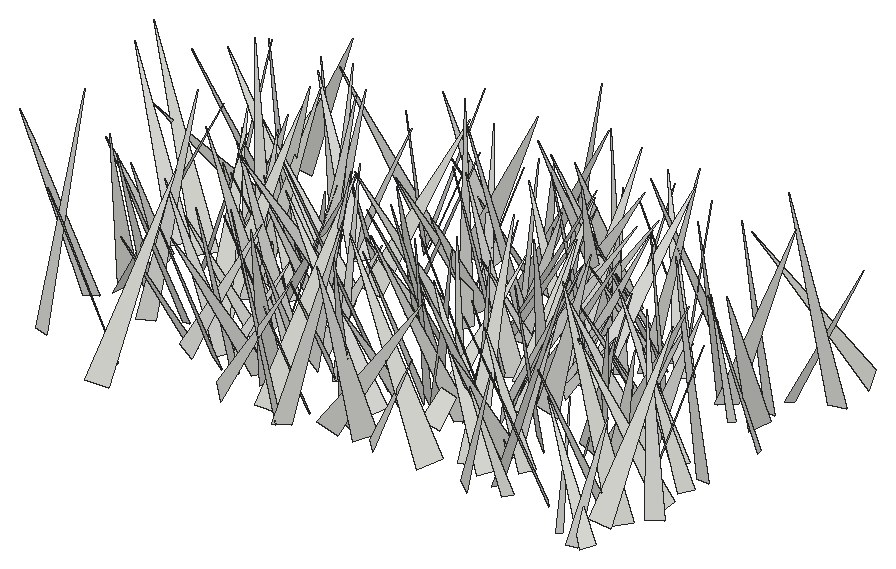
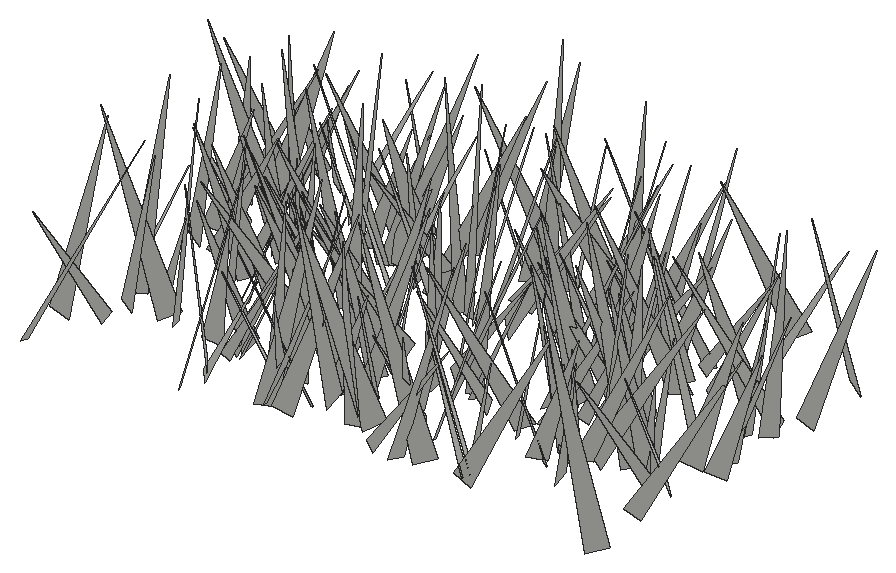
# SketchUp Ruby script. Lengths in inches.
U = 1.inch
M = Sketchup.active_model
def pt(a) = Geom::Point3d.new(a.map { |v| v * U })
def face(e, loops, mat)
  f = e.add_face(loops[0].map { |a| pt(a) })
  loops[1..].each { |l| e.add_face(l.map { |a| pt(a) }).erase! }
  f.material = f.back_material = mat if mat
  f
end
# faces: each face lists its corners as indices into pts; further lists are holes
def faces(e, pts, list, mat = nil) = list.each { |f| face(e, (f[0].is_a?(Array) ? f : [f]).map { |l| l.map { |i| pts[i] } }, mat) }
# xy, xz, yz: faces in a plane at the given z, y or x. An outline is a flat list of corners, or four numbers for a rectangle; further outlines are holes
def ring(l) = l.size == 4 ? [[l[0], l[1]], [l[2], l[1]], [l[2], l[3]], [l[0], l[3]]] : l.each_slice(2).to_a
def flat(e, list, mat, &to3) = list.each { |f| face(e, (f[0].is_a?(Array) ? f : [f]).map { |l| ring(l).map { |u, v| to3.(u, v) } }, mat) }
def xy(e, z, list, mat = nil) = flat(e, list, mat) { |x, y| [x, y, z] }
def xz(e, y, list, mat = nil) = flat(e, list, mat) { |x, z| [x, y, z] }
def yz(e, x, list, mat = nil) = flat(e, list, mat) { |y, z| [x, y, z] }
def lines(e, pts, list) = list.each { |a, b| e.add_line(pt(pts[a]), pt(pts[b])) }
# prism: a flat outline (further loops are holes) pulled along v
def prism(e, loops, v, mat = nil)
  f = face(e, loops, mat); d = Geom::Vector3d.new(v.map { |x| x * U })
  f.pushpull(f.normal.samedirection?(d) ? d.length : -d.length)
end
def box(e, o, s, mat = nil) = prism(e, [[o, [o[0] + s[0], o[1], o[2]], [o[0] + s[0], o[1] + s[1], o[2]], [o[0], o[1] + s[1], o[2]]]], [0, 0, s[2]], mat)
def at(x, y, z, deg = 0) = Geom::Transformation.translation(pt([x, y, z])) * Geom::Transformation.rotation(ORIGIN, Z_AXIS, deg.degrees)
def axes(o, x, y, z) = Geom::Transformation.new([*x, 0, *y, 0, *z, 0, *pt(o).to_a, 1])
def part(name) = M.definitions.add(name)
# library, detail: a bought-in or finely detailed component or shape, given as its bounding box
def library(name, o, s) = part(name).tap { |d| box(d.entities, o, s) }
def detail(e, o, s) = box(e.add_group.entities, o, s)
def put(e, d, t, mat = nil) = e.add_instance(d, t).tap { |i| i.material = mat if mat }
def group(e, t, mat = nil) = e.add_group.tap { |g| g.transformation = t; g.material = mat if mat }.entities
root = M.entities
c1 = part("fur_instance\#9")
p = [[0.8125,0,1.79],[0.67,-0.02,1.48],[0,-0.11,0],[0,0.11,0]]
faces(c1.entities,p,[[0,1,2,3]])
put(root,c1,axes([479.78,414.29,-21.66],[5.20163,-5.29224,1.8402],[-4.95757,-5.51713,-1.85336],[-2.61089,-0.0677,7.18539]))
put(root,c1,axes([461.92,409.04,-21.66],[-4.61251,5.93847,1.25396],[5.3205,4.71401,-2.75381],[2.92064,0.79104,6.99694]))
put(root,c1,axes([478.12,414.66,-21.66],[-1.25565,-8.18969,1.33935],[-8.04493,1.53362,1.83538],[2.03567,1.00923,8.07955]))
put(root,c1,axes([461.29,411.97,-21.66],[-4.82792,-3.85999,0.34861],[-3.62589,4.30173,-2.58417],[-1.36894,2.21934,5.6152]))
put(root,c1,axes([468.7,413.11,-21.66],[4.45492,4.83666,0.95124],[4.56601,-3.56591,-3.25273],[1.85733,-2.83468,5.71483]))
put(root,c1,axes([488.74,413.21,-21.66],[3.06956,3.90435,1.71137],[4.25532,-2.68017,-1.51785],[0.25498,-2.27325,4.72887]))
put(root,c1,axes([499.9,412,-21.66],[-3.00277,4.1066,0.06153],[3.92812,2.84936,1.52829],[-1.19912,-0.94951,4.85234]))
put(root,c1,axes([474.04,412.49,-21.66],[-6.46812,-3.13785,1.21731],[-3.3431,6.29489,-1.53709],[0.38946,1.92167,7.02282]))
put(root,c1,axes([466.18,416.07,-21.66],[-2.99336,-6.46525,0.18966],[-6.30073,2.9619,1.52434],[1.46161,-0.47255,6.9596]))
put(root,c1,axes([499.04,411.47,-21.66],[-3.77654,1.99621,0.89861],[1.50689,3.67022,-1.82025],[1.58796,1.26459,3.86442]))
put(root,c1,axes([477.2,413.66,-21.66],[3.63581,-6.29578,1.08718],[-5.74464,-2.67402,3.72648],[2.79605,2.69271,6.24254]))
put(root,c1,axes([480.76,413.72,-21.66],[2.90459,3.11145,0.76807],[3.13189,-2.53582,-1.57117],[0.67994,-1.61126,3.9559]))
put(root,c1,axes([470.27,416.52,-21.66],[7.22069,-3.00234,1.05262],[-2.62839,-7.10035,-2.22196],[-1.79266,-1.6827,7.49769]))
put(root,c1,axes([491.67,414.07,-21.66],[-1.39517,3.65073,1.37856],[3.73252,0.82124,1.60268],[-1.13865,-1.78115,3.56451]))
put(root,c1,axes([485.2,414.16,-21.66],[-7.15301,3.97515,0.71331],[4.02795,6.91641,1.848],[-0.2937,-1.95899,7.97197]))
put(root,c1,axes([469.38,416.59,-21.66],[1.60402,-6.13136,0.73735],[-5.58582,-1.76536,-2.52831],[-2.63361,0.00991,5.81155]))
put(root,c1,axes([497.26,412.36,-21.66],[1.37607,4.21587,0.41156],[3.82506,-1.42264,1.78368],[-1.81985,0.19763,4.06025]))
put(root,c1,axes([494.35,414.9,-21.66],[-5.23491,-4.53939,0.15815],[-4.43832,5.06084,-1.65066],[-0.96564,1.34804,6.72946]))
put(root,c1,axes([474.78,414.67,-21.66],[-4.9499,-5.12629,0.49866],[-4.98162,4.58947,-2.26921],[-1.30806,1.92014,6.75508]))
put(root,c1,axes([474.51,412.32,-21.66],[6.67924,-1.26552,2.75336],[-2.18749,-6.62541,2.26131],[-2.097,2.88046,6.41095]))
put(root,c1,axes([498.57,415.85,-21.66],[-1.67937,-5.43767,0.87836],[-5.25266,1.30456,-1.96667],[-1.65811,1.37475,5.34049]))
put(root,c1,axes([454.89,412.18,-21.66],[3.59561,7.30217,1.1805],[7.09033,-3.77639,1.76345],[-2.10771,-0.24675,7.94609]))
put(root,c1,axes([488.53,418.25,-21.66],[5.3138,-2.81187,1.14067],[-1.98861,-4.96443,-2.9739],[-2.29198,-2.2118,5.22484]))
put(root,c1,axes([488.16,417.92,-21.66],[-0.28332,-7.79704,0.77926],[-7.68212,0.12267,-1.56569],[-1.54472,0.82004,7.64347]))
put(root,c1,axes([463.92,416.53,-21.66],[-1.49578,-4.28811,0.26565],[-3.87905,1.22698,-2.03551],[-1.84701,0.89578,4.0598]))
put(root,c1,axes([478.81,419.45,-21.66],[-5.2943,-3.28141,1.0592],[-2.29433,4.80125,3.40634],[2.57403,-2.46971,5.21479]))
put(root,c1,axes([472.74,419.83,-21.66],[-3.72735,-5.65721,0.3773],[-4.71825,3.34531,3.54775],[3.14396,-1.68653,5.77153]))
put(root,c1,axes([467.91,415.76,-21.66],[-2.85535,-4.62994,1.75531],[-4.89429,2.33192,-1.81068],[-0.75056,2.40755,5.12941]))
put(root,c1,axes([488.83,415.6,-21.66],[-4.99082,4.3261,0.4502],[4.29852,4.80129,1.51542],[-0.66378,-1.43477,6.4286]))
put(root,c1,axes([499.73,415.64,-21.66],[-2.9065,7.574,1.65107],[7.44857,2.24028,2.83534],[-2.14716,-2.4809,7.60092]))
put(root,c1,axes([471.26,418.73,-21.66],[-5.10979,-2.8974,1.28802],[-2.4355,5.15064,1.92434],[2.03034,-1.11347,5.54994]))
put(root,c1,axes([463.72,415.92,-21.66],[1.55014,5.60518,1.20615],[5.3228,-0.94254,-2.46072],[2.13086,-1.72318,5.26933]))
put(root,c1,axes([466.02,417.1875,-21.66],[-3.70212,4.89762,1.86065],[5.19102,3.12087,2.11373],[-0.70854,-2.72541,5.76407]))
put(root,c1,axes([454.44,417.83,-21.66],[-0.79345,-6.87819,1.77521],[-6.83318,0.25089,-2.08208],[-1.94125,1.92821,6.60333]))
put(root,c1,axes([490.68,417.3,-21.66],[-3.29735,3.76242,1.32483],[3.9802,2.99017,1.41439],[-0.2628,-1.92005,4.79874]))
put(root,c1,axes([498.5625,414.88,-21.66],[-1.75958,6.89289,0.89816],[6.66639,1.93582,-1.79628],[1.96924,-0.39424,6.88342]))
put(root,c1,axes([472.59,413.27,-21.66],[-6.00676,5.62271,0.83771],[4.81686,5.68135,-3.59416],[3.01902,2.12255,7.40122]))
put(root,c1,axes([490.35,414.62,-21.66],[7.12647,2.20024,1.82821],[1.44023,-6.99989,2.8102],[-2.47167,2.26505,6.90872]))
put(root,c1,axes([500.64,419.2,-21.66],[-6.49837,1.01991,0.13564],[1.01971,6.26851,1.71854],[-0.13717,-1.71841,6.34946]))
put(root,c1,axes([483.36,419.9375,-21.66],[0.24896,-7.3468,1.55373],[-6.97419,-0.80255,-2.67734],[-2.78393,1.35351,6.84612]))
put(root,c1,axes([468.35,418.7,-21.66],[-2.5232,4.5633,1.53247],[4.25008,1.29942,3.12842],[-2.26029,-2.65076,4.17172]))
put(root,c1,axes([466.23,417.38,-21.66],[1.55212,3.88569,0.28277],[3.69063,-1.36892,-1.44671],[1.24813,-0.78428,3.92616]))
put(root,c1,axes([479.39,420.81,-21.66],[-5.06426,-4.56399,0.84014],[-4.29824,5.08189,1.69768],[1.74956,-0.72593,6.60262]))
put(root,c1,axes([478.31,417.26,-21.66],[-3.77529,6.85051,0.02559],[5.94676,3.26269,3.89536],[-3.40091,-1.89957,6.78296]))
put(root,c1,axes([480.08,420.4,-21.66],[-3.33298,-6.74445,1.96036],[-6.484,3.7887,2.01069],[2.69971,0.77298,7.24938]))
put(root,c1,axes([461.41,418.87,-21.66],[-3.32714,-4.87132,0.7615],[-4.7527,2.92423,-2.05917],[-1.31203,1.7603,5.52806]))
put(root,c1,axes([489.04,420.68,-21.66],[-3.9717,-6.10655,1.7462],[-5.81347,4.32471,1.90107],[2.55787,0.34722,7.03209]))
put(root,c1,axes([488.62,418.5,-21.66],[-0.11529,-4.79427,2.44231],[-5.06003,0.9271,1.58106],[1.8292,2.26244,4.52754]))
put(root,c1,axes([480.81,420.27,-21.66],[7.66875,0.29762,1.40281],[0.64374,-7.5341,-1.92071],[-1.28143,-2.00373,7.43029]))
put(root,c1,axes([455.2,420.63,-21.66],[6.33398,-2.31725,1.64534],[-1.9481,-6.46653,-1.60778],[-2.06922,-1.00519,6.55011]))
put(root,c1,axes([456.36,421.3125,-21.66],[6.05103,1.03829,2.78411],[2.19851,-5.8136,-2.61017],[-1.99898,-3.2509,5.55698]))
put(root,c1,axes([501.05,417.45,-21.66],[-0.8728,6.82324,1.17968],[6.78553,0.6058,1.51645],[-1.38016,-1.33658,6.7096]))
put(root,c1,axes([486.65,419.37,-21.66],[-5.69424,-4.56861,0.52497],[-4.47673,5.31586,-2.29625],[-1.05201,2.10752,6.92992]))
put(root,c1,axes([493.01,421.88,-21.66],[-1.64763,-7.14584,1.34901],[-6.49832,2.06763,3.01567],[3.26416,0.50931,6.68457]))
put(root,c1,axes([466.42,421.19,-21.66],[-7.9399,0.37328,2.34081],[0.92834,8.01881,1.87016],[2.18103,-2.05426,7.72553]))
put(root,c1,axes([487.23,415.73,-21.66],[-7.03666,4.34174,0.35439],[3.96979,6.66848,-2.87454],[1.79361,2.2741,7.75256]))
put(root,c1,axes([491.99,421.95,-21.66],[0.44147,-7.17503,0.62576],[-6.54369,-0.13768,3.03788],[3.00878,0.75334,6.51516]))
put(root,c1,axes([471.04,419.7,-21.66],[-2.12698,-6.60371,3.80122],[-7.1046,3.14508,1.48842],[2.75369,3.0136,6.77625]))
put(root,c1,axes([477.26,419.98,-21.66],[-5.76145,-5.93812,0.42997],[-5.44241,5.01036,-3.73055],[-2.41379,2.87671,7.38502]))
put(root,c1,axes([468.77,420.61,-21.66],[-0.03383,-6.90938,2.82252],[-7.12958,-0.80509,-2.05628],[-2.20801,2.70547,6.5964]))
put(root,c1,axes([485.42,418.86,-21.66],[-5.55203,-0.57439,2.02149],[-1.15794,5.60149,-1.58866],[1.75372,1.88009,5.3508]))
put(root,c1,axes([494.51,421.6,-21.66],[1.53942,-5.44162,0.89342],[-5.38829,-1.28703,1.44538],[1.17292,1.22946,5.46735]))
put(root,c1,axes([459.17,417.55,-21.66],[-6.96616,2.88196,1.8212],[2.05018,6.85162,-3.00033],[2.72382,2.21349,6.91601]))
put(root,c1,axes([493.77,421.69,-21.66],[6.6749,-4.96789,0.00129],[-4.8195,-6.47499,2.02019],[1.20515,1.62135,8.07174]))
put(root,c1,axes([463.91,418.66,-21.66],[-5.45003,5.37343,0.92209],[5.18096,5.51046,-1.48977],[1.69756,0.43353,7.50714]))
put(root,c1,axes([482.04,418.16,-21.66],[-1.93127,6.17376,0.09606],[5.65668,1.80943,-2.5656],[2.47519,0.68189,5.93825]))
put(root,c1,axes([500.32,421.61,-21.66],[-2.9134,4.03937,1.46912],[4.26943,2.51447,1.5531],[-0.49677,-2.07934,4.73205]))
put(root,c1,axes([484.7,422.12,-21.66],[7.11507,4.33314,0.48127],[4.20256,-6.57141,-2.9643],[1.16029,-2.76992,7.78545]))
put(root,c1,axes([470.51,421.43,-21.66],[0.36945,4.73641,1.83647],[4.53767,0.52011,-2.25427],[2.28381,-1.79961,4.18191]))
put(root,c1,axes([455.34,419.4,-21.66],[7.33228,1.89466,0.16833],[1.78282,-7.07911,2.02191],[-0.66303,1.91751,7.29821]))
put(root,c1,axes([477.05,425.04,-21.66],[-6.01376,-4.74049,2.00405],[-3.98095,6.23797,2.80955],[3.26197,-1.12665,7.12348]))
put(root,c1,axes([473.85,419,-21.66],[2.20032,6.76237,0.49836],[6.15454,-2.21163,2.83722],[-2.84601,0.44546,6.52083]))
put(root,c1,axes([463.13,419.77,-21.66],[-0.97355,8.05143,1.14446],[7.84551,1.23329,-2.00251],[2.14086,-0.85824,7.85896]))
put(root,c1,axes([498.41,419.92,-21.66],[4.22042,3.02936,0.44277],[2.70703,-4.0447,1.87014],[-1.43005,1.2839,4.84681]))
put(root,c1,axes([495.32,423.91,-21.66],[-6.50951,0.22142,0.60358],[0.38251,6.26967,1.82536],[0.51674,-1.85181,6.25226]))
put(root,c1,axes([483.3,420.03,-21.66],[5.52585,4.05046,1.31825],[3.69086,-5.63091,1.83015],[-2.12639,0.75214,6.60241]))
put(root,c1,axes([468.01,420.34,-21.66],[4.5765,3.32185,0.66717],[3.07667,-4.544,1.52],[-1.41913,0.86116,5.4469]))
put(root,c1,axes([468.84,426.58,-21.66],[-7.67561,-3.02253,0.64542],[-2.50236,7.09168,3.4516],[1.81396,-3.00659,7.49247]))
put(root,c1,axes([454.91,424.7,-21.66],[-4.32761,-0.50237,2.11035],[0.41917,4.42689,1.9134],[2.12844,-1.89326,3.91401]))
put(root,c1,axes([481.89,421.5,-21.66],[1.02305,5.31057,1.33507],[5.15193,-1.39366,1.59576],[-1.8553,-0.94167,5.16743]))
put(root,c1,axes([455.43,424.59,-21.66],[-5.22696,-1.19875,0.73288],[-0.94186,5.08442,1.59898],[1.04259,-1.41663,5.11873]))
put(root,c1,axes([484.66,423.32,-21.66],[6.0574,2.72005,0.2303],[2.69232,-5.86042,-1.5971],[0.45071,-1.54939,6.44516]))
put(root,c1,axes([458.29,424.24,-21.66],[6.75177,1.95337,0.7466],[2.07523,-6.56983,-1.57805],[-0.25785,-1.72661,6.84922]))
put(root,c1,axes([486.82,424.2,-21.66],[1.53835,-7.01276,2.03333],[-7.04829,-0.88366,2.28484],[1.90652,2.39168,6.80623]))
put(root,c1,axes([481.24,425.9,-21.66],[-2.96228,-3.48582,0.87467],[-2.85625,2.97145,2.16874],[2.18125,-0.843,4.02773]))
put(root,c1,axes([500.28,423.32,-21.66],[1.97558,6.78512,3.04566],[6.89111,-2.85534,1.89119],[-2.79761,-2.24188,6.80913]))
put(root,c1,axes([492.22,421.23,-21.66],[4.15865,3.49208,0.81847],[2.77358,-3.92559,2.6563],[-2.27416,1.59814,4.73636]))
put(root,c1,axes([462.6,427.25,-21.66],[-3.43989,-5.36661,0.1848],[-4.97328,3.26677,2.29397],[2.02515,-1.09328,5.94736]))
put(root,c1,axes([485.08,426.16,-21.66],[-0.53699,-7.34105,1.16615],[-7.27133,0.76139,1.44476],[1.5423,1.0337,7.21748]))
put(root,c1,axes([497.86,424.13,-21.66],[-2.44299,5.49091,1.30941],[5.27932,1.71736,2.64808],[-1.99837,-2.17564,5.395]))
put(root,c1,axes([465.14,423.4375,-21.66],[5.97099,-0.01983,0.33196],[-0.11666,-5.7151,1.75709],[-0.31141,1.76085,5.70664]))
put(root,c1,axes([492.93,427.53,-21.66],[-4.66281,-2.88259,0.04543],[-2.761,4.48988,1.50703],[0.82963,-1.25893,5.27068]))
put(root,c1,axes([473.41,428.08,-21.66],[-0.94018,-7.50089,0.47804],[-7.29693,1.02641,1.75419],[1.80188,0.24278,7.35324]))
put(root,c1,axes([484.875,424.46,-21.66],[6.3813,-2.25892,0.20905],[-2.20352,-6.02357,2.17449],[0.53935,2.11689,6.41056]))
put(root,c1,axes([492.47,425.29,-21.66],[3.58397,-3.64133,0.7361],[-3.60405,-3.15993,1.91614],[0.90107,1.84433,4.7363]))
put(root,c1,axes([465.87,426.41,-21.66],[0.12283,-4.44104,1.09952],[-4.1986,-0.54638,-1.73783],[-1.81756,0.96203,4.08875]))
put(root,c1,axes([462.5,423.79,-21.66],[4.91626,-1.03874,2.91243],[-2.03601,-5.20453,1.58061],[-2.3272,2.35896,4.76972]))
put(root,c1,axes([492.23,427.76,-21.66],[-3.17214,-2.54983,0.51656],[-2.07776,2.97317,1.9168],[1.56569,-1.22048,3.59026]))
put(root,c1,axes([494.35,425.24,-21.66],[3.63193,-4.05591,1.60644],[-4.34601,-3.18259,1.79036],[0.37856,2.37544,5.14159]))
put(root,c1,axes([485.71,423.1,-21.66],[-4.47907,3.89554,0.463],[3.44419,4.24137,-2.36643],[1.87807,1.51235,5.44401]))
put(root,c1,axes([467.35,424.28,-21.66],[-6.57541,3.25527,2.97746],[2.73361,7.20101,-1.83599],[3.46258,0.49673,7.10365]))
put(root,c1,axes([486.16,426.7,-21.66],[2.45066,3.05169,0.44917],[2.65928,-1.79957,-2.28257],[1.56295,-1.7231,3.17938]))
put(root,c1,axes([465.07,425.48,-21.66],[-1.27036,4.00789,0.19304],[3.62684,1.0603,1.85365],[-1.71652,-0.72583,3.77372]))
put(root,c1,axes([476.07,426.9375,-21.66],[-2.89235,-4.23355,0.19447],[-3.82387,2.50545,-2.32964],[-1.82723,1.45817,4.56743]))
put(root,c1,axes([482.33,426.53,-21.66],[0.18988,-6.4583,3.19895],[-6.79344,-1.22898,-2.07794],[-2.40669,2.95955,6.11783]))
put(root,c1,axes([473.21,428.62,-21.66],[-4.08154,-1.42978,0.42723],[-1.12455,3.76494,1.85644],[0.98091,-1.633,3.906]))
put(root,c1,axes([481.54,426.43,-21.66],[-6.3033,-3.29184,1.05702],[-3.45211,6.11366,-1.54635],[0.19083,1.86335,6.94094]))
put(root,c1,axes([474.08,429.76,-21.66],[-6.53247,-2.60599,0.49941],[-2.30056,6.22381,2.3844],[1.32211,-2.04617,6.61657]))
put(root,c1,axes([468.03,424.8125,-21.66],[2.36714,6.37429,1.14743],[6.22522,-2.57637,1.46983],[-1.78738,-0.5313,6.63886]))
put(root,c1,axes([485.68,426.96,-21.66],[2.51119,2.94201,0.30611],[2.79372,-2.22715,-1.51331],[0.97173,-1.19981,3.55969]))
put(root,c1,axes([482.82,428.89,-21.66],[-4.59731,-1.23154,0.33008],[-1.08177,4.4213,1.42926],[0.67485,-1.30242,4.53973]))
put(root,c1,axes([458.12,429.05,-21.66],[4.10212,-1.60455,0.85508],[-1.23063,-4.00368,-1.60913],[-1.3384,-1.23658,4.10033]))
put(root,c1,axes([467.38,428.17,-21.66],[-6.03456,2.61232,0.13904],[2.52964,5.73798,1.98392],[-0.66667,-1.87372,6.2693]))
put(root,c1,axes([461.77,425.67,-21.66],[6.32729,-2.1008,2.73388],[-3.01636,-6.1404,2.26257],[-1.67006,3.13117,6.27127]))
put(root,c1,axes([462.29,425.95,-21.66],[0.0482,8.00911,1.76337],[7.92916,-0.49572,2.03478],[-2.09374,-1.69294,7.74648]))
put(root,c1,axes([454.68,426.76,-21.66],[-3.24359,5.98487,0.42852],[5.75195,2.96279,2.1587],[-1.708,-1.38792,6.45597]))
put(root,c1,axes([456.8,426.6875,-21.66],[-3.17251,7.14398,0.8627],[6.87917,2.73438,2.65436],[-2.11131,-1.82544,7.35225]))
put(root,c1,axes([459.48,429.16,-21.66],[3.88235,-7.18309,1.19208],[-7.15051,-3.50623,2.16032],[1.37403,2.04942,7.87416]))
put(root,c1,axes([494.06,427.4375,-21.66],[-3.8782,-4.63911,2.52217],[-5.26639,3.62608,-1.42825],[0.38461,2.87286,5.87554]))
put(root,c1,axes([498.68,431.16,-21.66],[5.9537,-4.05045,0.58701],[-3.75603,-5.81897,-2.05648],[-1.62572,-1.38951,6.90098]))
put(root,c1,axes([463.2,427.6,-21.66],[-7.60319,-2.30719,2.08818],[-2.71089,7.61771,-1.45385],[1.52798,2.03457,7.8114]))
put(root,c1,axes([483.4,425.94,-21.66],[-1.05391,6.67902,0.37292],[6.52998,1.10912,-1.41007],[1.4518,-0.14015,6.613]))
put(root,c1,axes([458.13,429.19,-21.66],[3.9818,-4.86666,0.84742],[-4.90357,-3.76221,1.43455],[0.59785,1.55519,6.12218]))
put(root,c1,axes([500.71,428.59,-21.66],[-4.67684,-2.75,0.36196],[-2.71074,4.38122,-1.73872],[-0.58771,1.67594,5.13928]))
put(root,c1,axes([475.25,431.89,-21.66],[4.02503,-3.95124,0.17731],[-3.62061,-3.78264,-2.10414],[-1.59215,-1.38705,5.23314]))
put(root,c1,axes([480.17,426.38,-21.66],[6.45135,0.1489,0.38361],[-0.04006,-5.77049,2.9136],[-0.40954,2.91007,5.75787]))
put(root,c1,axes([484.93,429.23,-21.66],[5.1253,5.35023,0.94765],[5.22805,-4.50107,-2.86349],[1.48003,-2.62814,6.83331]))
put(root,c1,axes([467.77,430.71,-21.66],[-3.99319,-2.60087,1.40659],[-2.16034,4.18012,1.59628],[2.0189,-0.6713,4.49021]))
put(root,c1,axes([459.36,427.92,-21.66],[-0.27528,4.26527,0.41219],[4.05575,0.12601,1.40472],[-1.38323,-0.47937,4.03672]))
put(root,c1,axes([462.17,429.875,-21.66],[-3.051,-7.21191,1.32168],[-6.61753,2.09219,-3.8598],[-3.15701,2.58422,6.81338]))
put(root,c1,axes([479.49,428.26,-21.66],[7.04502,0.38941,0.11832],[0.34745,-6.82295,1.76766],[-0.21195,1.75889,6.83077]))
put(root,c1,axes([462.61,430.52,-21.66],[-6.95314,3.37085,0.59923],[3.40426,6.66259,2.02209],[-0.36434,-2.07731,7.45788]))
put(root,c1,axes([479.64,430.24,-21.66],[3.48254,-4.50934,1.30252],[-4.66936,-3.1635,1.53235],[0.47726,1.95368,5.48763]))
put(root,c1,axes([462.06,431.64,-21.66],[-0.71595,-3.844,0.50308],[-3.36107,0.87042,1.86752],[1.93201,0.08975,3.4353]))
put(root,c1,axes([485.99,429.8,-21.66],[-6.23091,-2.8217,1.23434],[-3.03851,6.08694,-1.42355],[0.50305,1.81577,6.69027]))
put(root,c1,axes([455.6875,434.03,-21.66],[3.04305,-5.48081,0.27728],[-4.42438,-2.6378,-3.58374],[-3.24669,-1.54241,5.14356]))
put(root,c1,axes([481.29,430.38,-21.66],[4.41498,5.25807,0.18984],[4.81628,-3.93899,-2.90917],[2.11822,-2.00311,6.21901]))
put(root,c1,axes([479.53,431.31,-21.66],[-2.64388,-6.79077,2.11498],[-6.99476,2.07362,-2.08599],[-1.28885,2.67645,6.98236]))
put(root,c1,axes([471.73,434.27,-21.66],[-4.9139,-3.74374,0.55427],[-3.15126,4.55055,2.79845],[2.0958,-1.9355,5.50733]))
put(root,c1,axes([494.1875,432.79,-21.66],[-6.11732,-3.75265,2.76683],[-3.28898,6.70851,1.82699],[3.3046,-0.26993,6.94018]))
put(root,c1,axes([475.89,429.49,-21.66],[-7.47088,0.3057,1.86762],[-0.12287,7.51123,-1.721],[1.88848,1.69808,7.27638]))
put(root,c1,axes([463.24,431.3,-21.66],[2.35807,6.09522,2.44102],[6.53945,-1.94795,-1.45322],[0.58808,-2.77931,6.37184]))
put(root,c1,axes([471.66,428.73,-21.66],[5.28462,2.45266,0.54887],[2.09175,-5.00051,2.20534],[-1.39334,1.79538,5.39252]))
put(root,c1,axes([496.86,430.56,-21.66],[0.33091,4.05955,1.18914],[3.81261,-0.80293,1.68011],[-1.83248,-0.93747,3.71034]))
put(root,c1,axes([483.33,434.07,-21.66],[6.57894,-4.30915,0.69378],[-4.10201,-6.53322,-1.6802],[-1.49116,-1.03963,7.68298]))
put(root,c1,axes([488.18,433.6,-21.66],[-4.30266,-2.43803,0.04686],[-2.30354,4.09498,1.544],[0.79994,-1.32144,4.69819]))
put(root,c1,axes([468.21,429.34,-21.66],[-2.47927,6.31853,1.78834],[5.49074,3.04318,-3.14001],[3.60191,-0.28983,6.01756]))
put(root,c1,axes([487.06,428.09,-21.66],[-2.37553,7.32496,0.20013],[6.77476,2.27563,-2.87444],[2.79244,0.71043,7.14393]))
put(root,c1,axes([489.23,433.16,-21.66],[-2.79932,-5.24784,0.26282],[-5.09915,2.64134,-1.57068],[-1.26789,0.96362,5.73663]))
put(root,c1,axes([479.86,432.33,-21.66],[5.30447,3.34271,0.68413],[3.37643,-4.96043,-1.94241],[0.49141,-1.99988,5.96139]))
put(root,c1,axes([479.98,432.875,-21.66],[3.5795,-7.50714,1.0436],[-6.77337,-2.6505,4.166],[3.40115,2.62237,7.19823]))
put(root,c1,axes([484.29,429.32,-21.66],[-4.73234,6.09922,1.47861],[5.53404,4.92888,-2.61961],[2.95993,0.53615,7.26177]))
put(root,c1,axes([464.15,432.39,-21.66],[4.41432,4.17138,0.78555],[4.1779,-4.06951,-1.86761],[0.75011,-1.88212,5.77916]))
put(root,c1,axes([495.09,432.25,-21.66],[6.69732,-3.52244,1.21858],[-3.71872,-6.48437,1.69431],[-0.25228,2.07171,7.37503]))
put(root,c1,axes([456.86,430.49,-21.66],[-1.28039,5.01222,0.36244],[4.5705,1.31696,-2.06622],[2.08908,0.19072,4.74262]))
put(root,c1,axes([456.03,429.87,-21.66],[3.80784,5.11048,0.67094],[4.57882,-3.73693,2.47721],[-2.36675,0.99257,5.87197]))
put(root,c1,axes([463.74,430.95,-21.66],[1.51119,6.34193,0.92742],[6.21067,-1.68435,1.39797],[-1.58356,-0.55387,6.36784]))
put(root,c1,axes([489,434.17,-21.66],[-0.33006,-3.76044,0.39687],[-3.50265,0.15395,-1.45434],[-1.42474,0.49269,3.4835]))
put(root,c1,axes([465.05,432.16,-21.66],[-4.13597,4.87198,0.25098],[4.78591,3.98836,1.44689],[-0.94567,-1.12348,6.22487]))
put(root,c1,axes([487.36,431.03,-21.66],[-7.91635,-0.39433,1.24518],[-0.80795,7.48837,-2.76517],[1.02625,2.85367,7.42819]))
put(root,c1,axes([498.09,432.92,-21.66],[1.91991,5.69676,2.84026],[5.7974,-2.78995,1.67703],[-2.62873,-1.9923,5.77292]))
put(root,c1,axes([478.6,431.75,-21.66],[2.37609,4.94692,0.8109],[4.47755,-2.49789,2.11838],[-2.25414,0.25283,5.06264]))
put(root,c1,axes([480.75,433.375,-21.66],[-2.13288,4.47426,0.69403],[4.36785,1.83113,1.61826],[-1.19274,-1.2953,4.68502]))
put(root,c1,axes([483.03,437.55,-21.66],[6.13444,-4.45258,1.42838],[-3.84619,-6.14459,-2.6359],[-2.65943,-1.38408,7.10696]))
put(root,c1,axes([462.23,433.27,-21.66],[-5.98582,-0.44068,0.88109],[-0.67667,5.78235,-1.70504],[0.71598,1.78068,5.75475]))
put(root,c1,axes([488.52,432.16,-21.66],[6.48387,0.57283,2.72889],[-0.5216,-6.53637,2.61139],[-2.73914,2.60063,5.96233]))
put(root,c1,axes([483.16,437.07,-21.66],[-6.61379,-2.13915,0.88077],[-1.88588,6.53057,1.69974],[1.33985,-1.36736,6.74011]))
put(root,c1,axes([477.05,436.13,-21.66],[-0.17668,-5.97479,1.5156],[-5.97573,0.53792,1.42395],[1.51188,1.4279,5.80532]))
put(root,c1,axes([473.65,432.85,-21.66],[3.6245,2.89722,0.22495],[2.66528,-3.45765,1.58821],[-1.15791,1.11007,4.35987]))
put(root,c1,axes([481.72,437.46,-21.66],[0.79588,-7.21699,0.96951],[-7.03929,-1.01213,-1.75565],[-1.86367,0.74092,7.04528]))
put(root,c1,axes([475.84,435.28,-21.66],[7.56022,-3.29271,0.03526],[-3.23696,-7.41517,1.59297],[0.60437,1.47429,8.09082]))
put(root,c1,axes([490.92,433.15,-21.66],[-1.83761,6.5724,0.07775],[6.30696,1.74042,1.94227],[-1.85059,-0.59481,6.54223]))
put(root,c1,axes([480.63,435.76,-21.66],[4.14208,3.82367,0.06036],[3.46383,-3.71363,-2.44781],[1.62049,-1.8356,5.07794]))
put(root,c1,axes([470.43,436.875,-21.66],[3.82613,-7.13137,0.63835],[-6.75778,-3.35774,2.99351],[2.36564,1.94225,7.51895]))
put(root,c1,axes([500.92,436.34,-21.66],[-1.04276,-7.37455,2.60053],[-7.71345,0.53914,-1.56404],[-1.28435,2.74945,7.28184]))
put(root,c1,axes([467.01,437.32,-21.66],[-0.65869,-6.64833,1.3688],[-6.16249,0.00919,-2.92087],[-2.84565,1.51902,6.00855]))
put(root,c1,axes([467.14,436.91,-21.66],[4.68379,1.41709,0.13919],[1.37897,-4.39495,-1.65779],[0.35492,-1.62533,4.60411]))
put(root,c1,axes([488.79,439.15,-21.66],[-6.12859,-4.53414,1.24355],[-3.97845,6.08997,2.59781],[2.50535,-1.42065,7.16724]))
put(root,c1,axes([488.38,436.73,-21.66],[5.36268,3.16176,1.79895],[3.56295,-5.21159,-1.4615],[-0.73371,-2.1986,6.05138]))
put(root,c1,axes([474.11,433.75,-21.66],[0.39127,5.5531,0.09038],[5.24022,-0.39914,1.8382],[-1.83989,0.04412,5.25462]))
put(root,c1,axes([479.92,434.33,-21.66],[-7.4216,0.05563,3.73189],[-0.80703,8.0859,-1.72548],[3.64401,1.90407,7.21845]))
put(root,c1,axes([472.16,437.78,-21.66],[-6.75805,0.02177,1.99006],[0.56326,6.77748,1.83863],[1.90881,-1.92284,6.50317]))
put(root,c1,axes([467.12,436.24,-21.66],[6.01088,3.96881,0.98389],[4.08835,-5.80352,-1.56674],[0.06989,-1.84874,7.03046]))
put(root,c1,axes([467.625,435.58,-21.66],[1.94279,3.86541,2.10519],[3.74501,-2.66073,1.42935],[-2.3126,-1.06149,4.08323]))
put(root,c1,axes([485.15,434.02,-21.66],[3.44077,4.42208,0.21812],[4.18127,-3.33634,1.68138],[-1.45578,0.8691,5.34478]))
put(root,c1,axes([474.41,437.58,-21.66],[-2.08934,-4.39389,0.06996],[-3.98317,1.86084,-2.08523],[-1.85622,0.95264,4.39584]))
put(root,c1,axes([483.43,435.2,-21.66],[-4.4668,1.24969,0.75909],[0.98308,4.37301,-1.41442],[1.08236,1.18546,4.4174]))
put(root,c1,axes([500.48,440.5,-21.66],[-7.29463,-2.71144,0.02018],[-2.47986,6.69465,3.09773],[1.09665,-2.89718,7.13916]))
put(root,c1,axes([498.13,434.97,-21.66],[5.03908,0.51167,0.65236],[0.18588,-4.61324,2.18248],[-0.80798,2.12978,4.57066]))
put(root,c1,axes([454.51,439.1,-21.66],[3.10816,-7.62871,0.22312],[-7.12075,-2.81203,3.04879],[2.74626,1.34273,7.65263]))
put(root,c1,axes([488.52,436.97,-21.66],[-3.99392,-3.16377,0.39905],[-3.06383,3.62986,-1.88605],[-0.88412,1.71311,4.73326]))
